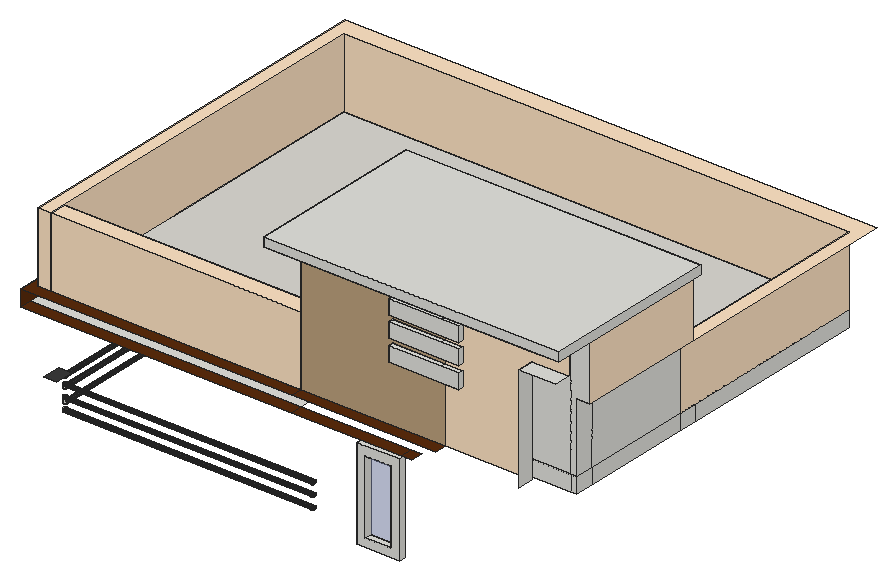
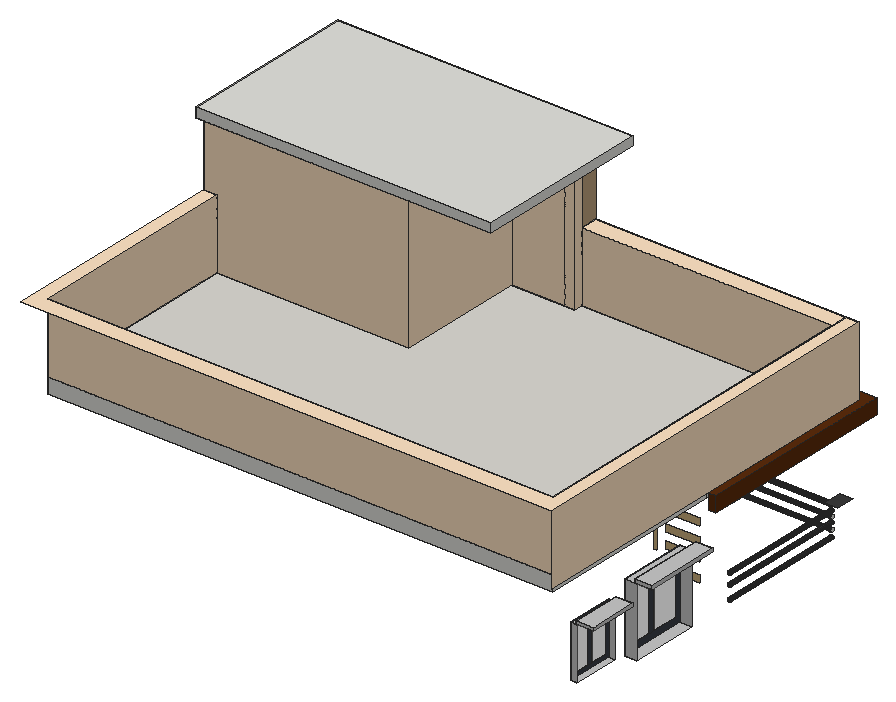
# SketchUp Ruby script. Lengths in inches.
U = 1.inch
M = Sketchup.active_model
def pt(a) = Geom::Point3d.new(a.map { |v| v * U })
def face(e, loops, mat)
  f = e.add_face(loops[0].map { |a| pt(a) })
  loops[1..].each { |l| e.add_face(l.map { |a| pt(a) }).erase! }
  f.material = f.back_material = mat if mat
  f
end
# faces: each face lists its corners as indices into pts; further lists are holes
def faces(e, pts, list, mat = nil) = list.each { |f| face(e, (f[0].is_a?(Array) ? f : [f]).map { |l| l.map { |i| pts[i] } }, mat) }
# xy, xz, yz: faces in a plane at the given z, y or x. An outline is a flat list of corners, or four numbers for a rectangle; further outlines are holes
def ring(l) = l.size == 4 ? [[l[0], l[1]], [l[2], l[1]], [l[2], l[3]], [l[0], l[3]]] : l.each_slice(2).to_a
def flat(e, list, mat, &to3) = list.each { |f| face(e, (f[0].is_a?(Array) ? f : [f]).map { |l| ring(l).map { |u, v| to3.(u, v) } }, mat) }
def xy(e, z, list, mat = nil) = flat(e, list, mat) { |x, y| [x, y, z] }
def xz(e, y, list, mat = nil) = flat(e, list, mat) { |x, z| [x, y, z] }
def yz(e, x, list, mat = nil) = flat(e, list, mat) { |y, z| [x, y, z] }
def lines(e, pts, list) = list.each { |a, b| e.add_line(pt(pts[a]), pt(pts[b])) }
# prism: a flat outline (further loops are holes) pulled along v
def prism(e, loops, v, mat = nil)
  f = face(e, loops, mat); d = Geom::Vector3d.new(v.map { |x| x * U })
  f.pushpull(f.normal.samedirection?(d) ? d.length : -d.length)
end
def box(e, o, s, mat = nil) = prism(e, [[o, [o[0] + s[0], o[1], o[2]], [o[0] + s[0], o[1] + s[1], o[2]], [o[0], o[1] + s[1], o[2]]]], [0, 0, s[2]], mat)
def at(x, y, z, deg = 0) = Geom::Transformation.translation(pt([x, y, z])) * Geom::Transformation.rotation(ORIGIN, Z_AXIS, deg.degrees)
def axes(o, x, y, z) = Geom::Transformation.new([*x, 0, *y, 0, *z, 0, *pt(o).to_a, 1])
def part(name) = M.definitions.add(name)
# library, detail: a bought-in or finely detailed component or shape, given as its bounding box
def library(name, o, s) = part(name).tap { |d| box(d.entities, o, s) }
def detail(e, o, s) = box(e.add_group.entities, o, s)
def put(e, d, t, mat = nil) = e.add_instance(d, t).tap { |i| i.material = mat if mat }
def group(e, t, mat = nil) = e.add_group.tap { |g| g.transformation = t; g.material = mat if mat }.entities
root = M.entities
M.materials.add("[0012_Bisque]").color = [255, 228, 196]
M.materials.add("[0035_Tan]").color = [188, 161, 125]
M.materials.add("[0043_SaddleBrown]").color = [91, 44, 12]
M.materials.add("[Color M02]").color = [198, 198, 198]
M.materials.add("[Color M07]").color = [58, 58, 58]
M.materials.add("[Formica Beige]").color = [211, 187, 149]
M.materials.add("[Formica Laminate Dark]").color = [59, 63, 71]
M.materials.add("[Terrazzo Tile Light]").color = [219, 217, 210]
M.materials.add("[Translucent Glass Gray]").color = [128, 128, 128]
M.materials["[Translucent Glass Gray]"].alpha = 0.5
M.materials.add("[Translucent Glass Sky Reflection]").color = [126, 138, 183]
M.materials["[Translucent Glass Sky Reflection]"].alpha = 0.52
M.materials.add("[Wood Cherry Original]").color = [89, 50, 24]
M.materials.add("[Wood Floor Light]").color = [204, 176, 127]
xy(root,769.18,[[378.07,387.15,418.25,393.34]])
xy(root,771.97,[[73.92,589.12,85.11,653.81]],"[Color M02]")
xy(root,777.375,[[386.26,387.15,410.06,393.34]])
xy(root,777.72,[[201.38,538.2,265.3,554.26]],"[Formica Beige]")
xy(root,784.22,[[73.92,679.68,79.48,723.8]],"[Color M02]")
xy(root,791.0625,[[173.82,407.81,174.21,407.86,174.57,408.01,174.88,408.25,175.12,408.56,175.27,408.92,175.32,409.31,175.27,409.7,175.12,410.06,174.88,410.37,174.57,410.61,174.21,410.76,173.82,410.81,173.43,410.76,173.07,410.61,172.76,410.37,172.52,410.06,172.37,409.7,172.32,409.31,172.37,408.92,172.52,408.56,172.76,408.25,173.07,408.01,173.43,407.86]])
xy(root,791.5625,[[275.5,407.81,275.89,407.86,276.25,408.01,276.57,408.25,276.8,408.56,276.95,408.92,277,409.31,276.95,409.7,276.8,410.06,276.57,410.37,276.25,410.61,275.89,410.76,275.5,410.81,275.12,410.76,274.75,410.61,274.44,410.37,274.21,410.06,274.06,409.7,274,409.31,274.06,408.92,274.21,408.56,274.44,408.25,274.75,408.01,275.12,407.86]])
xy(root,791.57,[[223,407.81,223.39,407.86,223.75,408.01,224.07,408.25,224.3,408.56,224.45,408.92,224.5,409.31,224.45,409.7,224.3,410.06,224.07,410.37,223.75,410.61,223.63,410.66,222.38,410.66,222.25,410.61,221.94,410.37,221.71,410.06,221.56,409.7,221.5,409.31,221.56,408.92,221.71,408.56,221.94,408.25,222.25,408.01,222.62,407.86],[222.38,410.66,223.63,410.66,223.39,410.76,223,410.81,222.62,410.76]])
xy(root,792.02,[[127.44,407.81,127.83,407.86,128.19,408.01,128.5,408.25,128.74,408.56,128.89,408.92,128.94,409.31,128.89,409.7,128.74,410.06,128.5,410.37,128.2,410.6,126.68,410.6,126.38,410.37,126.14,410.06,125.99,409.7,125.94,409.31,125.99,408.92,126.14,408.56,126.38,408.25,126.69,408.01,127.05,407.86],[126.68,410.6,128.2,410.6,128.19,410.61,127.83,410.76,127.44,410.81,127.05,410.76,126.69,410.61]])
xy(root,792.3125,[[79.17,509.6,79.5625,509.65,79.92,509.8,80.23,510.04,80.47,510.35,80.62,510.71,80.67,511.1,80.62,511.49,80.47,511.85,80.23,512.16,79.92,512.4,79.5625,512.55,79.17,512.6,78.78,512.55,78.42,512.4,78.11,512.16,77.875,511.85,77.72,511.49,77.67,511.1,77.72,510.71,77.875,510.35,78.11,510.04,78.42,509.8,78.78,509.65]])
xy(root,792.5625,[[79.17,436.29,79.5625,436.34,79.92,436.49,80.23,436.73,80.47,437.04,80.62,437.4,80.67,437.79,80.62,438.18,80.47,438.54,80.23,438.85,79.92,439.09,79.5625,439.24,79.17,439.29,78.78,439.24,78.42,439.09,78.11,438.85,77.875,438.54,77.72,438.18,77.67,437.79,77.72,437.4,77.875,437.04,78.11,436.73,78.42,436.49,78.78,436.34]])
xy(root,793.125,[[79.17,472.66,79.5625,472.72,79.92,472.87,80.23,473.1,80.47,473.41,80.62,473.78,80.67,474.16,80.62,474.55,80.47,474.91,80.23,475.23,79.92,475.46,79.5625,475.61,79.17,475.66,78.78,475.61,78.42,475.46,78.11,475.23,77.875,474.91,77.72,474.55,77.67,474.16,77.72,473.78,77.875,473.41,78.11,473.1,78.42,472.87,78.78,472.72]])
xy(root,796.5,[[73.92,401.01,85.98,418.04]],"[Color M07]")
xy(root,832.97,[[73.92,679.68,79.48,723.8]],"[Color M02]")
xy(root,833.97,[[57.67,678.66,73.92,725.11]],"[Color M02]")
xy(root,836.66,[[73.92,589.12,85.11,653.81],[57.67,678.66,73.92,725.11]],"[Color M02]")
xy(root,838.57,[[57.67,584.97,73.92,656.41]],"[Color M02]")
xy(root,841.76,[[57.67,584.97,73.92,656.41]],"[Color M02]")
xy(root,846.36,[[386.26,387.15,410.06,393.34]])
xy(root,846.97,[[201.38,538.2,265.3,554.26]],"[Formica Beige]")
xy(root,854.55,[[378.07,387.15,418.25,393.34]])
xy(root,861.625,[[66.61,393.34,66.61,538.2,560.26,538.2,560.26,418.04,320.99,418.04,320.99,393.34],[85.98,538.2,560.26,556.28],[85.98,556.28,560.26,737.09]])
xy(root,861.625,[[66.61,382.09,320.99,393.34],[320.99,382.09,424.43,393.34],[424.43,382.09,434.25,393.34],[66.61,538.2,73.92,569.95]],"[0043_SaddleBrown]")
xy(root,876.375,[[73.92,393.34,85.98,538.2],[85.98,393.34,320.99,409.47],[379.95,418.04,560.26,538.2]])
xy(root,876.375,[[66.61,382.09,320.99,382.09,320.99,393.34,73.92,393.34,73.92,569.95,66.61,569.95],[320.99,382.09,456.39,393.34]],"[0043_SaddleBrown]")
xy(root,876.375,[[85.98,409.47,320.99,409.47,320.99,418.04,379.95,418.04,379.95,538.2,560.26,538.2,560.26,737.09,85.98,737.09]],"[Terrazzo Tile Light]")
xy(root,931.66,[[406.9,388.72,456.39,393.34],[456.39,388.72,472.72,393.34]])
xy(root,941.875,[[560.26,418.04,572.32,434.85],[560.26,434.85,572.32,538.2]])
xy(root,941.875,[[73.92,393.34,85.98,393.34,85.98,737.09,560.26,737.09,560.26,538.2,572.32,538.2,572.32,753.91,73.92,753.91],[85.98,393.34,320.99,409.47]],"[0012_Bisque]")
xy(root,945.53,[[406.9,388.72,456.39,393.34],[456.39,388.72,472.72,393.34]])
xy(root,951.66,[[406.9,388.72,456.39,393.34],[456.39,388.72,472.72,393.34]])
xy(root,965.53,[[406.9,388.72,456.39,393.34],[456.39,388.72,472.72,393.34]])
xy(root,971.1,[[406.9,388.72,456.39,393.34],[456.39,388.72,472.72,393.34]])
xy(root,975.8,[[537.68,378.34,572.32,393.34]])
xy(root,984.97,[[406.9,388.72,456.39,393.34],[456.39,388.72,472.72,393.34]])
xy(root,999.875,[[303.81,371.66,303.81,393.34,537.68,393.34,554.62,371.66],[554.62,371.66,537.68,393.34,580.07,393.34,580.07,371.66],[303.81,393.34,320.99,409.47],[320.99,393.34,537.68,393.34,554.62,418.04,320.99,418.04],[537.68,393.34,572.32,393.34,572.32,418.04,554.62,418.04],
  [572.32,393.34,580.07,418.04],[303.81,409.47,320.99,418.04],[303.81,418.04,379.95,538.2],[379.95,418.04,572.32,538.2],[572.32,418.04,580.07,538.2]])
xy(root,1008.4375,[[303.81,371.66,580.07,538.2]])
xz(root,371.66,[[303.81,999.875,580.07,1008.4375]])
xz(root,387.15,[[[378.07,769.18,418.25,854.55],[386.26,777.375,410.06,846.36]]])
xz(root,388.72,[[406.9,931.66,472.72,945.53],[406.9,951.66,472.72,965.53],[406.9,971.1,472.72,984.97]])
xz(root,393.34,[[[378.07,769.18,418.25,854.55],[386.26,777.375,410.06,846.36]],[406.9,931.66,472.72,945.53],[406.9,951.66,472.72,965.53],[406.9,971.1,472.72,984.97]])
xz(root,393.34,[[73.92,876.375,85.98,941.875],[85.98,876.375,320.99,941.875],[456.39,876.375,537.68,876.375,537.68,975.8,572.32,975.8,572.32,999.875,456.39,999.875,456.39,984.97,472.72,984.97,472.72,971.1,456.39,971.1,456.39,965.53,472.72,965.53,472.72,951.66,456.39,951.66,456.39,945.53,472.72,945.53,472.72,931.66,456.39,931.66]],"[0012_Bisque]")
xz(root,393.34,[[320.99,876.375,456.39,876.375,456.39,931.66,406.9,931.66,406.9,945.53,456.39,945.53,456.39,951.66,406.9,951.66,406.9,965.53,456.39,965.53,456.39,971.1,406.9,971.1,406.9,984.97,456.39,984.97,456.39,999.875,320.99,999.875]],"[0035_Tan]")
xz(root,393.34,[[386.26,777.375,410.06,846.36]],"[Translucent Glass Sky Reflection]")
xz(root,409.47,[[85.98,876.375,320.99,941.875]],"[0012_Bisque]")
xz(root,418.04,[[79.68,768.35,80.13,768.41,80.55,768.58,80.91,768.86,81.19,769.22,81.37,769.64,81.43,770.1,81.37,770.55,81.19,770.97,80.91,771.33,80.55,771.61,80.13,771.79,79.68,771.85,79.22,771.79,78.8,771.61,78.4375,771.33,78.16,770.97,77.99,770.55,77.93,770.1,77.99,769.64,78.16,769.22,78.4375,768.86,78.8,768.58,79.22,768.41],[79.68,781.03,80.13,781.09,80.55,781.27,80.91,781.55,81.19,781.91,81.37,782.33,81.43,782.78,81.37,783.24,81.19,783.66,80.91,784.02,80.55,784.3,80.13,784.47,79.68,784.53,79.22,784.47,78.8,784.3,78.4375,784.02,78.16,783.66,77.99,783.24,77.93,782.78,77.99,782.33,78.16,781.91,78.4375,781.55,78.8,781.27,79.22,781.09],[79.68,790.85,80.13,790.91,80.55,791.08,80.91,791.36,81.19,791.72,81.37,792.14,81.43,792.6,81.37,793.05,81.19,793.47,80.91,793.83,80.55,794.11,80.13,794.29,79.68,794.35,79.22,794.29,78.8,794.11,78.4375,793.83,78.16,793.47,77.99,793.05,77.93,792.6,77.99,792.14,78.16,791.72,78.4375,791.36,78.8,791.08,79.22,790.91],[320.99,861.625,329.72,876.375],[329.72,861.625,554.62,876.375],
  [554.62,861.625,560.26,876.375],[379.95,876.375,554.62,999.875],[554.62,876.375,554.62,999.875,572.32,999.875,572.32,941.875,560.26,941.875,560.26,876.375]])
xz(root,418.04,[[320.99,876.375,329.72,999.875],[329.72,876.375,379.95,999.875]],"[0012_Bisque]")
xz(root,538.2,[[303.81,999.875,580.07,1008.4375]])
xz(root,538.2,[[379.95,876.375,379.95,999.875,572.32,999.875,572.32,941.875,560.26,941.875,560.26,876.375]],"[0012_Bisque]")
xz(root,538.2,[[107.76,774.27,138.82,781.34],[147.39,788.3,150.51,806.24],[107.76,792.02,138.82,799.09],[107.76,806.52,138.82,813.59],[107.76,822.27,138.82,829.34]],"[Wood Floor Light]")
xz(root,554.26,[[[201.38,777.72,265.3,846.97],[205.86,782.19,260.83,842.5]],[205.86,782.19,231.1,842.5],[231.1,782.19,236.78,842.5],[236.78,782.19,260.83,842.5]],"[Wood Cherry Original]")
xz(root,569.95,[[66.61,861.625,73.92,876.375]],"[0043_SaddleBrown]")
xz(root,584.97,[[57.67,838.57,73.92,841.76]],"[Color M02]")
xz(root,589.12,[[73.92,771.97,85.11,836.66]],"[Color M02]")
xz(root,653.81,[[73.92,771.97,85.11,836.66]],"[Color M02]")
xz(root,656.41,[[57.67,838.57,73.92,841.76]],"[Color M02]")
xz(root,678.66,[[57.67,833.97,73.92,836.66]],"[Color M02]")
xz(root,679.68,[[73.92,784.22,79.48,832.97]],"[Color M02]")
xz(root,723.8,[[73.92,784.22,79.48,832.97]],"[Color M02]")
xz(root,725.11,[[57.67,833.97,73.92,836.66]],"[Color M02]")
xz(root,737.09,[[85.98,861.625,560.26,876.375]])
xz(root,737.09,[[85.98,876.375,560.26,941.875]],"[0012_Bisque]")
yz(root,57.67,[[678.66,833.97,725.11,836.66],[584.97,838.57,656.41,841.76]],"[Color M02]")
yz(root,66.61,[[382.09,861.625,569.95,876.375]],"[0043_SaddleBrown]")
yz(root,73.92,[[678.66,833.97,725.11,836.66],[584.97,838.57,656.41,841.76]])
yz(root,73.92,[[393.34,876.375,753.91,941.875]],"[0012_Bisque]")
yz(root,79.48,[[[679.68,784.22,723.8,832.97],[683.63,788.17,719.85,829.02]],[700.07,788.17,704.29,829.02]],"[Formica Laminate Dark]")
yz(root,79.48,[[683.63,788.17,700.07,829.02],[704.29,788.17,719.85,829.02]],"[Translucent Glass Gray]")
yz(root,85.11,[[[589.12,771.97,653.81,836.66],[594.7,777.55,648.23,831.08]],[619.4375,777.55,625.43,831.08]],"[Formica Laminate Dark]")
yz(root,85.11,[[594.7,777.55,619.4375,831.08],[625.43,777.55,648.23,831.08]],"[Translucent Glass Gray]")
yz(root,85.98,[[408.91,768.38,408.45,768.44,408.03,768.62,407.67,768.9,407.39,769.26,407.22,769.68,407.16,770.13,407.22,770.59,407.39,771.01,407.67,771.37,408.03,771.65,408.45,771.82,408.91,771.88,409.36,771.82,409.78,771.65,410.14,771.37,410.42,771.01,410.6,770.59,410.66,770.13,410.6,769.68,410.42,769.26,410.14,768.9,409.78,768.62,409.36,768.44],[408.91,779.13,408.45,779.19,408.03,779.37,407.67,779.65,407.39,780.01,407.22,780.43,407.16,780.88,407.22,781.34,407.39,781.76,407.67,782.12,408.03,782.4,408.45,782.57,408.91,782.63,409.36,782.57,409.78,782.4,410.14,782.12,410.42,781.76,410.6,781.34,410.66,780.88,410.6,780.43,410.42,780.01,410.14,779.65,409.78,779.37,409.36,779.19],[408.91,789.82,408.45,789.88,408.03,790.06,407.67,790.33,407.39,790.7,407.22,791.12,407.16,791.57,407.22,792.02,407.39,792.45,407.67,792.81,408.03,793.09,408.45,793.26,408.91,793.32,409.36,793.26,409.78,793.09,410.14,792.81,410.42,792.45,410.6,792.02,410.66,791.57,410.6,791.12,410.42,790.7,410.14,790.33,409.78,790.06,409.36,789.88],[538.2,861.625,556.28,876.375],[556.28,861.625,737.09,876.375],
  [393.34,876.375,409.47,941.875]])
yz(root,85.98,[[409.47,876.375,737.09,941.875]],"[0012_Bisque]")
yz(root,201.38,[[538.2,777.72,554.26,846.97]],"[Formica Beige]")
yz(root,265.3,[[538.2,777.72,554.26,846.97]],"[Formica Beige]")
yz(root,303.81,[[371.66,999.875,538.2,1008.4375]])
yz(root,320.99,[[393.34,876.375,409.47,941.875]])
yz(root,320.99,[[409.47,876.375,418.04,999.875]],"[0012_Bisque]")
yz(root,320.99,[[393.34,941.875,409.47,999.875]],"[0035_Tan]")
yz(root,378.07,[[387.15,769.18,393.34,854.55]])
yz(root,379.95,[[418.04,876.375,538.2,999.875]],"[0012_Bisque]")
yz(root,386.26,[[387.15,777.375,393.34,846.36]])
yz(root,406.9,[[388.72,931.66,393.34,945.53],[388.72,951.66,393.34,965.53],[388.72,971.1,393.34,984.97]])
yz(root,410.06,[[387.15,777.375,393.34,846.36]])
yz(root,418.25,[[387.15,769.18,393.34,854.55]])
yz(root,472.72,[[388.72,931.66,393.34,945.53],[388.72,951.66,393.34,965.53],[388.72,971.1,393.34,984.97]])
yz(root,537.68,[[378.34,876.375,393.34,975.8]])
yz(root,560.26,[[418.04,861.625,434.85,876.375],[434.85,861.625,538.2,876.375],[538.2,861.625,556.28,876.375],[556.28,861.625,737.09,876.375],[418.04,876.375,434.85,941.875],
  [434.85,876.375,538.2,941.875]])
yz(root,560.26,[[538.2,876.375,737.09,941.875]],"[0012_Bisque]")
yz(root,572.32,[[418.04,941.875,538.2,999.875]],"[0012_Bisque]")
yz(root,580.07,[[371.66,999.875,538.2,1008.4375]])
p = [[79.68,418.04,768.35],[79.22,418.04,768.41],[79.22,538.2,768.41],[79.68,538.2,768.35],[80.13,418.04,768.41],[80.13,538.2,768.41],
  [85.98,408.03,768.62],[85.98,408.45,768.44],[320.99,408.45,768.44],[320.99,408.03,768.62],[85.98,408.91,768.38],[320.99,408.91,768.38],
  [85.98,409.36,768.44],[320.99,409.36,768.44],[85.98,409.78,768.62],[320.99,409.78,768.62],[78.8,418.04,768.58],[78.8,538.2,768.58],
  [80.55,418.04,768.58],[80.55,538.2,768.58],[85.98,407.67,768.9],[320.99,407.67,768.9],[85.98,410.14,768.9],[320.99,410.14,768.9],
  [78.4375,418.04,768.86],[78.4375,538.2,768.86],[80.91,418.04,768.86],[80.91,538.2,768.86],[85.98,407.39,769.26],[320.99,407.39,769.26],
  [85.98,410.42,769.26],[320.99,410.42,769.26],[78.16,418.04,769.22],[78.16,538.2,769.22],[81.19,418.04,769.22],[81.19,538.2,769.22],
  [77.99,418.04,769.64],[77.99,538.2,769.64],[81.37,418.04,769.64],[81.37,538.2,769.64],[85.98,407.22,769.68],[320.99,407.22,769.68],
  [85.98,410.6,769.68],[320.99,410.6,769.68],[77.93,418.04,770.1],[77.93,538.2,770.1],[81.43,418.04,770.1],[81.43,538.2,770.1],
  [85.98,407.16,770.13],[320.99,407.16,770.13],[85.98,410.66,770.13],[320.99,410.66,770.13],[85.98,407.22,770.59],[320.99,407.22,770.59],
  [85.98,410.6,770.59],[320.99,410.6,770.59],[77.99,418.04,770.55],[77.99,538.2,770.55],[81.37,418.04,770.55],[81.37,538.2,770.55],
  [78.16,418.04,770.97],[78.16,538.2,770.97],[81.19,418.04,770.97],[81.19,538.2,770.97],[85.98,407.39,771.01],[320.99,407.39,771.01],
  [85.98,410.42,771.01],[320.99,410.42,771.01],[85.98,407.67,771.37],[320.99,407.67,771.37],[85.98,410.14,771.37],[320.99,410.14,771.37],
  [78.4375,418.04,771.33],[78.4375,538.2,771.33],[80.91,418.04,771.33],[80.91,538.2,771.33],[78.8,418.04,771.61],[78.8,538.2,771.61],
  [80.55,418.04,771.61],[80.55,538.2,771.61],[85.98,408.03,771.65],[320.99,408.03,771.65],[85.98,409.78,771.65],[320.99,409.78,771.65],
  [85.98,408.45,771.82],[320.99,408.45,771.82],[85.98,409.36,771.82],[320.99,409.36,771.82],[79.22,418.04,771.79],[79.22,538.2,771.79],
  [80.13,418.04,771.79],[80.13,538.2,771.79],[85.98,408.91,771.88],[320.99,408.91,771.88],[79.68,418.04,771.85],[79.68,538.2,771.85],
  [85.98,408.45,779.19],[85.98,408.91,779.13],[320.99,408.91,779.13],[320.99,408.45,779.19],[85.98,409.36,779.19],[320.99,409.36,779.19],
  [85.98,408.03,779.37],[320.99,408.03,779.37],[85.98,409.78,779.37],[320.99,409.78,779.37],[85.98,407.67,779.65],[320.99,407.67,779.65],
  [85.98,410.14,779.65],[320.99,410.14,779.65],[85.98,407.39,780.01],[320.99,407.39,780.01],[85.98,410.42,780.01],[320.99,410.42,780.01],
  [85.98,407.22,780.43],[320.99,407.22,780.43],[85.98,410.6,780.43],[320.99,410.6,780.43],[85.98,407.16,780.88],[320.99,407.16,780.88],
  [85.98,410.66,780.88],[320.99,410.66,780.88],[85.98,407.22,781.34],[320.99,407.22,781.34],[85.98,410.6,781.34],[320.99,410.6,781.34],
  [79.68,418.04,781.03],[79.22,418.04,781.09],[79.22,538.2,781.09],[79.68,538.2,781.03],[80.13,418.04,781.09],[80.13,538.2,781.09],
  [78.8,418.04,781.27],[78.8,538.2,781.27],[80.55,418.04,781.27],[80.55,538.2,781.27],[85.98,407.39,781.76],[320.99,407.39,781.76],
  [85.98,410.42,781.76],[320.99,410.42,781.76],[78.4375,418.04,781.55],[78.4375,538.2,781.55],[80.91,418.04,781.55],[80.91,538.2,781.55],
  [78.16,418.04,781.91],[78.16,538.2,781.91],[81.19,418.04,781.91],[81.19,538.2,781.91],[85.98,407.67,782.12],[320.99,407.67,782.12],
  [85.98,410.14,782.12],[320.99,410.14,782.12],[77.99,418.04,782.33],[77.99,538.2,782.33],[81.37,418.04,782.33],[81.37,538.2,782.33],
  [85.98,408.03,782.4],[320.99,408.03,782.4],[85.98,409.78,782.4],[320.99,409.78,782.4],[77.93,418.04,782.78],[77.93,538.2,782.78],
  [81.43,418.04,782.78],[81.43,538.2,782.78],[85.98,408.45,782.57],[320.99,408.45,782.57],[85.98,409.36,782.57],[320.99,409.36,782.57],
  [85.98,408.91,782.63],[320.99,408.91,782.63],[77.99,418.04,783.24],[77.99,538.2,783.24],[81.37,418.04,783.24],[81.37,538.2,783.24],
  [78.16,418.04,783.66],[78.16,538.2,783.66],[81.19,418.04,783.66],[81.19,538.2,783.66],[78.4375,418.04,784.02],[78.4375,538.2,784.02],
  [80.91,418.04,784.02],[80.91,538.2,784.02],[78.8,418.04,784.3],[78.8,538.2,784.3],[80.55,418.04,784.3],[80.55,538.2,784.3],
  [79.22,418.04,784.47],[79.22,538.2,784.47],[80.13,418.04,784.47],[80.13,538.2,784.47],[79.68,418.04,784.53],[79.68,538.2,784.53],
  [85.98,408.45,789.88],[85.98,408.91,789.82],[320.99,408.91,789.82],[320.99,408.45,789.88],[85.98,409.36,789.88],[320.99,409.36,789.88],
  [85.98,408.03,790.06],[320.99,408.03,790.06],[85.98,409.78,790.06],[320.99,409.78,790.06],[85.98,407.67,790.33],[320.99,407.67,790.33],
  [85.98,410.14,790.33],[320.99,410.14,790.33],[85.98,407.39,790.7],[320.99,407.39,790.7],[85.98,410.42,790.7],[320.99,410.42,790.7],
  [85.98,407.22,791.12],[320.99,407.22,791.12],[85.98,410.6,791.12],[320.99,410.6,791.12],[79.68,418.04,790.85],[79.22,418.04,790.91],
  [79.22,538.2,790.91],[79.68,538.2,790.85],[80.13,418.04,790.91],[80.13,538.2,790.91],[78.8,418.04,791.08],[78.8,538.2,791.08],
  [80.55,418.04,791.08],[80.55,538.2,791.08],[85.98,407.16,791.57],[320.99,407.16,791.57],[85.98,410.66,791.57],[222.38,410.66,791.57],
  [223.63,410.66,791.57],[320.99,410.66,791.57],[78.4375,418.04,791.36],[78.4375,538.2,791.36],[80.91,418.04,791.36],[80.91,538.2,791.36],
  [78.16,418.04,791.72],[78.16,538.2,791.72],[81.19,418.04,791.72],[81.19,538.2,791.72],[85.98,407.22,792.02],[320.99,407.22,792.02],
  [85.98,410.6,792.02],[126.68,410.6,792.02],[128.2,410.6,792.02],[320.99,410.6,792.02],[77.99,418.04,792.14],[77.99,538.2,792.14],
  [81.37,418.04,792.14],[81.37,538.2,792.14],[85.98,407.39,792.45],[320.99,407.39,792.45],[85.98,410.42,792.45],[320.99,410.42,792.45],
  [77.93,418.04,792.6],[77.93,538.2,792.6],[81.43,418.04,792.6],[81.43,538.2,792.6],[85.98,407.67,792.81],[320.99,407.67,792.81],
  [85.98,410.14,792.81],[320.99,410.14,792.81],[77.99,418.04,793.05],[77.99,538.2,793.05],[81.37,418.04,793.05],[81.37,538.2,793.05],
  [85.98,408.03,793.09],[320.99,408.03,793.09],[85.98,409.78,793.09],[320.99,409.78,793.09],[78.16,418.04,793.47],[78.16,538.2,793.47],
  [81.19,418.04,793.47],[81.19,538.2,793.47],[85.98,408.45,793.26],[320.99,408.45,793.26],[85.98,409.36,793.26],[320.99,409.36,793.26],
  [85.98,408.91,793.32],[320.99,408.91,793.32],[78.4375,418.04,793.83],[78.4375,538.2,793.83],[80.91,418.04,793.83],[80.91,538.2,793.83],
  [78.8,418.04,794.11],[78.8,538.2,794.11],[80.55,418.04,794.11],[80.55,538.2,794.11],[79.22,418.04,794.29],[79.22,538.2,794.29],
  [80.13,418.04,794.29],[80.13,538.2,794.29],[79.68,418.04,794.35],[79.68,538.2,794.35]]
faces(root,p,[[0,1,2,3],[4,0,3,5],[6,7,8,9],[7,10,11,8],[10,12,13,11],[12,14,15,13],[1,16,17,2],[18,4,5,19],
  [20,6,9,21],[14,22,23,15],[16,24,25,17],[26,18,19,27],[28,20,21,29],[22,30,31,23],[24,32,33,25],[34,26,27,35],
  [32,36,37,33],[38,34,35,39],[40,28,29,41],[30,42,43,31],[36,44,45,37],[46,38,39,47],[48,40,41,49],[42,50,51,43],
  [52,48,49,53],[50,54,55,51],[44,56,57,45],[58,46,47,59],[56,60,61,57],[62,58,59,63],[64,52,53,65],[54,66,67,55],
  [68,64,65,69],[66,70,71,67],[60,72,73,61],[74,62,63,75],[72,76,77,73],[78,74,75,79],[80,68,69,81],[70,82,83,71],
  [84,80,81,85],[82,86,87,83],[76,88,89,77],[90,78,79,91],[92,84,85,93],[86,92,93,87],[88,94,95,89],[94,90,91,95],
  [96,97,98,99],[97,100,101,98],[102,96,99,103],[100,104,105,101],[106,102,103,107],[104,108,109,105],[110,106,107,111],[108,112,113,109],
  [114,110,111,115],[112,116,117,113],[118,114,115,119],[116,120,121,117],[122,118,119,123],[120,124,125,121],[126,127,128,129],[130,126,129,131],
  [127,132,133,128],[134,130,131,135],[136,122,123,137],[124,138,139,125],[132,140,141,133],[142,134,135,143],[140,144,145,141],[146,142,143,147],
  [148,136,137,149],[138,150,151,139],[144,152,153,145],[154,146,147,155],[156,148,149,157],[150,158,159,151],[152,160,161,153],[162,154,155,163],
  [164,156,157,165],[158,166,167,159],[168,164,165,169],[166,168,169,167],[160,170,171,161],[172,162,163,173],[170,174,175,171],[176,172,173,177],
  [174,178,179,175],[180,176,177,181],[178,182,183,179],[184,180,181,185],[182,186,187,183],[188,184,185,189],[186,190,191,187],[190,188,189,191],
  [192,193,194,195],[193,196,197,194],[198,192,195,199],[196,200,201,197],[202,198,199,203],[200,204,205,201],[206,202,203,207],[204,208,209,205],
  [210,206,207,211],[208,212,213,209],[214,215,216,217],[218,214,217,219],[215,220,221,216],[222,218,219,223],[224,210,211,225],[212,226,227,228,229,213],
  [220,230,231,221],[232,222,223,233],[230,234,235,231],[236,232,233,237],[238,224,225,239],[226,240,241,242,243,229,228,227],[234,244,245,235],[246,236,237,247],
  [248,238,239,249],[240,250,251,243,242,241],[244,252,253,245],[254,246,247,255],[256,248,249,257],[250,258,259,251],[252,260,261,253],[262,254,255,263],
  [264,256,257,265],[258,266,267,259],[260,268,269,261],[270,262,263,271],[272,264,265,273],[266,274,275,267],[276,272,273,277],[274,276,277,275],
  [268,278,279,269],[280,270,271,281],[278,282,283,279],[284,280,281,285],[282,286,287,283],[288,284,285,289],[286,290,291,287],[290,288,289,291]],"[Color M07]")
